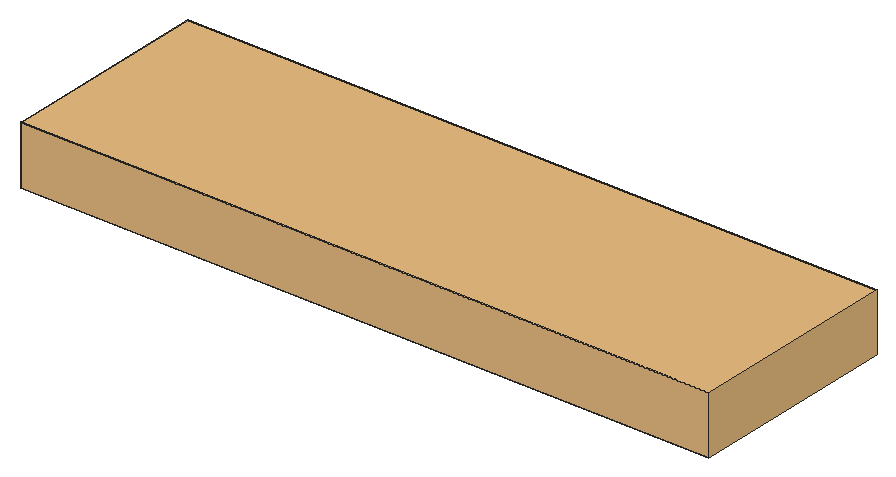
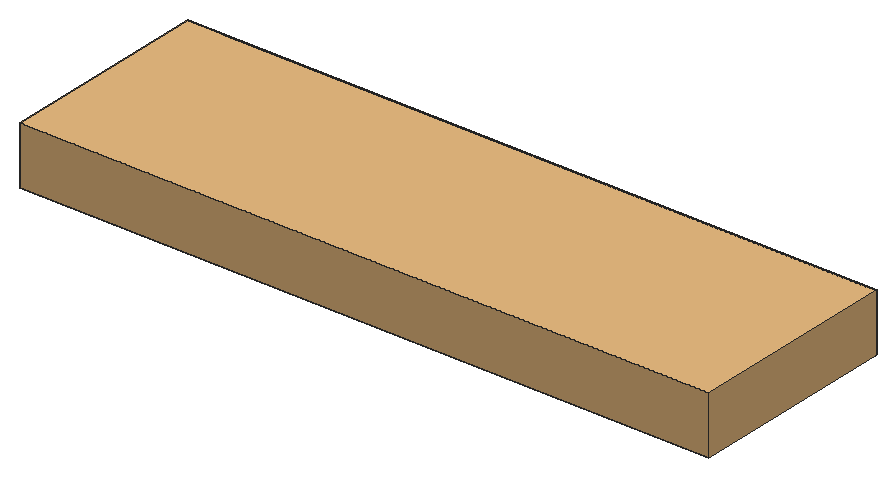
# SketchUp Ruby script. Lengths in inches.
U = 1.inch
M = Sketchup.active_model
def pt(a) = Geom::Point3d.new(a.map { |v| v * U })
def face(e, loops, mat)
  f = e.add_face(loops[0].map { |a| pt(a) })
  loops[1..].each { |l| e.add_face(l.map { |a| pt(a) }).erase! }
  f.material = f.back_material = mat if mat
  f
end
# faces: each face lists its corners as indices into pts; further lists are holes
def faces(e, pts, list, mat = nil) = list.each { |f| face(e, (f[0].is_a?(Array) ? f : [f]).map { |l| l.map { |i| pts[i] } }, mat) }
# xy, xz, yz: faces in a plane at the given z, y or x. An outline is a flat list of corners, or four numbers for a rectangle; further outlines are holes
def ring(l) = l.size == 4 ? [[l[0], l[1]], [l[2], l[1]], [l[2], l[3]], [l[0], l[3]]] : l.each_slice(2).to_a
def flat(e, list, mat, &to3) = list.each { |f| face(e, (f[0].is_a?(Array) ? f : [f]).map { |l| ring(l).map { |u, v| to3.(u, v) } }, mat) }
def xy(e, z, list, mat = nil) = flat(e, list, mat) { |x, y| [x, y, z] }
def xz(e, y, list, mat = nil) = flat(e, list, mat) { |x, z| [x, y, z] }
def yz(e, x, list, mat = nil) = flat(e, list, mat) { |y, z| [x, y, z] }
def lines(e, pts, list) = list.each { |a, b| e.add_line(pt(pts[a]), pt(pts[b])) }
# prism: a flat outline (further loops are holes) pulled along v
def prism(e, loops, v, mat = nil)
  f = face(e, loops, mat); d = Geom::Vector3d.new(v.map { |x| x * U })
  f.pushpull(f.normal.samedirection?(d) ? d.length : -d.length)
end
def box(e, o, s, mat = nil) = prism(e, [[o, [o[0] + s[0], o[1], o[2]], [o[0] + s[0], o[1] + s[1], o[2]], [o[0], o[1] + s[1], o[2]]]], [0, 0, s[2]], mat)
def at(x, y, z, deg = 0) = Geom::Transformation.translation(pt([x, y, z])) * Geom::Transformation.rotation(ORIGIN, Z_AXIS, deg.degrees)
def axes(o, x, y, z) = Geom::Transformation.new([*x, 0, *y, 0, *z, 0, *pt(o).to_a, 1])
def part(name) = M.definitions.add(name)
# library, detail: a bought-in or finely detailed component or shape, given as its bounding box
def library(name, o, s) = part(name).tap { |d| box(d.entities, o, s) }
def detail(e, o, s) = box(e.add_group.entities, o, s)
def put(e, d, t, mat = nil) = e.add_instance(d, t).tap { |i| i.material = mat if mat }
def group(e, t, mat = nil) = e.add_group.tap { |g| g.transformation = t; g.material = mat if mat }.entities
root = M.entities
M.materials.add("False ceiling Light").color = [253, 207, 127]
c1 = library("Group\#34",[0,0,-0.5],[272,74,0.5])
c2 = library("Group\#33",[0,-0.25,0],[284.26,86.25,24])
xz(root,214,[[99,228,368.95,252]])
xz(root,220,[[105,228,368.62,228.5]])
xz(root,221,[[106,228,368.56,228.5]])
xz(root,254,[[240.84,228,240.92,231],[240.92,228,241,231],[241,228,241.08,231],[241.08,228,241.16,231]])
xz(root,260,[[240.84,228,240.92,231],[240.92,228,241,231],[241,228,241.08,231],[241.08,228,241.16,231]])
xz(root,293,[[106,228,376,228.5]])
xz(root,294,[[105,228,377,228.5]])
yz(root,188,[[256.84,228,256.92,231],[256.92,228,257,231],[257,228,257.08,231],[257.08,228,257.16,231]])
yz(root,238,[[256.84,228,256.92,231],[256.92,228,257,231],[257,228,257.08,231],[257.08,228,257.16,231]])
yz(root,244,[[256.84,228,256.92,231],[256.92,228,257,231],[257,228,257.08,231],[257.08,228,257.16,231]])
yz(root,294,[[256.84,228,256.92,231],[256.92,228,257,231],[257,228,257.08,231],[257.08,228,257.16,231]])
p = [[240.53,254.04,228],[240.45,254.05,228],[240.45,254.05,231],[240.53,254.04,231],[240.61,254.03,228],[240.61,254.03,231],
  [240.6875,254.02,228],[240.6875,254.02,231],[240.76,254.01,228],[240.76,254.01,231],[240.84,254,228],[240.84,254,231],
  [241.24,254.01,228],[241.16,254,228],[241.16,254,231],[241.24,254.01,231],[241.3125,254.02,228],[241.3125,254.02,231],
  [241.39,254.03,228],[241.39,254.03,231],[241.47,254.04,228],[241.47,254.04,231],[241.55,254.05,228],[241.55,254.05,231],
  [240.07,254.15,228],[240,254.17,228],[240,254.17,231],[240.07,254.15,231],[240.15,254.125,228],[240.15,254.125,231],
  [240.22,254.1,228],[240.22,254.1,231],[240.3,254.08,228],[240.3,254.08,231],[240.375,254.07,228],[240.375,254.07,231],
  [241.625,254.07,228],[241.625,254.07,231],[241.7,254.08,228],[241.7,254.08,231],[241.78,254.1,228],[241.78,254.1,231],
  [241.85,254.125,228],[241.85,254.125,231],[241.93,254.15,228],[241.93,254.15,231],[242,254.17,228],[242,254.17,231],
  [186.22,254.26,228],[186.15,254.23,228],[186.15,254.23,231],[186.22,254.26,231],[239.85,254.23,228],[239.78,254.26,228],
  [239.78,254.26,231],[239.85,254.23,231],[239.92,254.2,228],[239.92,254.2,231],[242.08,254.2,228],[242.08,254.2,231],
  [242.15,254.23,228],[242.15,254.23,231],[242.22,254.26,228],[242.22,254.26,231],[186.29,254.29,228],[186.29,254.29,231],
  [186.36,254.33,228],[186.36,254.33,231],[186.43,254.36,228],[186.43,254.36,231],[239.64,254.33,228],[239.57,254.36,228],
  [239.57,254.36,231],[239.64,254.33,231],[239.71,254.29,228],[239.71,254.29,231],[242.29,254.29,228],[242.29,254.29,231],
  [242.36,254.33,228],[242.36,254.33,231],[242.43,254.36,228],[242.43,254.36,231],[186.5,254.4,228],[186.5,254.4,231],
  [186.57,254.44,228],[186.57,254.44,231],[186.63,254.48,228],[186.63,254.48,231],[239.43,254.44,228],[239.37,254.48,228],
  [239.37,254.48,231],[239.43,254.44,231],[239.5,254.4,228],[239.5,254.4,231],[242.5,254.4,228],[242.5,254.4,231],
  [242.57,254.44,228],[242.57,254.44,231],[242.63,254.48,228],[242.63,254.48,231],[186.7,254.53,228],[186.7,254.53,231],
  [186.76,254.57,228],[186.76,254.57,231],[239.3,254.53,228],[239.24,254.57,228],[239.24,254.57,231],[239.3,254.53,231],
  [242.7,254.53,228],[242.7,254.53,231],[242.76,254.57,228],[242.76,254.57,231],[186.83,254.62,228],[186.83,254.62,231],
  [186.89,254.67,228],[186.89,254.67,231],[239.17,254.62,228],[239.11,254.67,228],[239.11,254.67,231],[239.17,254.62,231],
  [242.83,254.62,228],[242.83,254.62,231],[242.89,254.67,228],[242.89,254.67,231],[186.95,254.72,228],[186.95,254.72,231],
  [187.01,254.77,228],[187.01,254.77,231],[239.05,254.72,228],[238.99,254.77,228],[238.99,254.77,231],[239.05,254.72,231],
  [242.95,254.72,228],[242.95,254.72,231],[243.01,254.77,228],[243.01,254.77,231],[187.07,254.82,228],[187.07,254.82,231],
  [187.12,254.88,228],[187.12,254.88,231],[238.93,254.82,228],[238.88,254.88,228],[238.88,254.88,231],[238.93,254.82,231],
  [243.07,254.82,228],[243.07,254.82,231],[243.12,254.88,228],[243.12,254.88,231],[187.18,254.93,228],[187.18,254.93,231],
  [187.23,254.99,228],[187.23,254.99,231],[238.82,254.93,228],[238.77,254.99,228],[238.77,254.99,231],[238.82,254.93,231],
  [243.18,254.93,228],[243.18,254.93,231],[243.23,254.99,228],[243.23,254.99,231],[187.28,255.05,228],[187.28,255.05,231],
  [238.72,255.05,228],[238.72,255.05,231],[243.28,255.05,228],[243.28,255.05,231],[294.77,254.99,228],[294.72,255.05,228],
  [294.72,255.05,231],[294.77,254.99,231],[187.33,255.11,228],[187.33,255.11,231],[187.38,255.17,228],[187.38,255.17,231],
  [238.67,255.11,228],[238.62,255.17,228],[238.62,255.17,231],[238.67,255.11,231],[243.33,255.11,228],[243.33,255.11,231],
  [243.38,255.17,228],[243.38,255.17,231],[294.67,255.11,228],[294.62,255.17,228],[294.62,255.17,231],[294.67,255.11,231],
  [187.43,255.24,228],[187.43,255.24,231],[187.47,255.3,228],[187.47,255.3,231],[238.57,255.24,228],[238.53,255.3,228],
  [238.53,255.3,231],[238.57,255.24,231],[243.43,255.24,228],[243.43,255.24,231],[243.47,255.3,228],[243.47,255.3,231],
  [294.57,255.24,228],[294.53,255.3,228],[294.53,255.3,231],[294.57,255.24,231],[187.52,255.37,228],[187.52,255.37,231],
  [238.48,255.37,228],[238.48,255.37,231],[243.52,255.37,228],[243.52,255.37,231],[294.48,255.37,228],[294.48,255.37,231],
  [187.56,255.43,228],[187.56,255.43,231],[187.6,255.5,228],[187.6,255.5,231],[238.44,255.43,228],[238.4,255.5,228],
  [238.4,255.5,231],[238.44,255.43,231],[243.56,255.43,228],[243.56,255.43,231],[243.6,255.5,228],[243.6,255.5,231],
  [294.44,255.43,228],[294.4,255.5,228],[294.4,255.5,231],[294.44,255.43,231],[187.64,255.57,228],[187.64,255.57,231],
  [238.36,255.57,228],[238.36,255.57,231],[243.64,255.57,228],[243.64,255.57,231],[294.36,255.57,228],[294.36,255.57,231],
  [187.67,255.64,228],[187.67,255.64,231],[187.71,255.71,228],[187.71,255.71,231],[238.33,255.64,228],[238.29,255.71,228],
  [238.29,255.71,231],[238.33,255.64,231],[243.67,255.64,228],[243.67,255.64,231],[243.71,255.71,228],[243.71,255.71,231],
  [294.33,255.64,228],[294.29,255.71,228],[294.29,255.71,231],[294.33,255.64,231],[187.74,255.78,228],[187.74,255.78,231],
  [238.26,255.78,228],[238.26,255.78,231],[243.74,255.78,228],[243.74,255.78,231],[294.26,255.78,228],[294.26,255.78,231],
  [187.77,255.85,228],[187.77,255.85,231],[238.23,255.85,228],[238.23,255.85,231],[243.77,255.85,228],[243.77,255.85,231],
  [294.23,255.85,228],[294.23,255.85,231],[187.8,255.92,228],[187.8,255.92,231],[187.83,256,228],[187.83,256,231],
  [238.2,255.92,228],[238.17,256,228],[238.17,256,231],[238.2,255.92,231],[243.8,255.92,228],[243.8,255.92,231],
  [243.83,256,228],[243.83,256,231],[294.2,255.92,228],[294.17,256,228],[294.17,256,231],[294.2,255.92,231],
  [187.85,256.07,228],[187.85,256.07,231],[238.15,256.07,228],[238.15,256.07,231],[243.85,256.07,228],[243.85,256.07,231],
  [294.15,256.07,228],[294.15,256.07,231],[187.875,256.15,228],[187.875,256.15,231],[187.9,256.22,228],[187.9,256.22,231],
  [238.125,256.15,228],[238.1,256.22,228],[238.1,256.22,231],[238.125,256.15,231],[243.875,256.15,228],[243.875,256.15,231],
  [243.9,256.22,228],[243.9,256.22,231],[294.125,256.15,228],[294.1,256.22,228],[294.1,256.22,231],[294.125,256.15,231],
  [187.92,256.3,228],[187.92,256.3,231],[238.08,256.3,228],[238.08,256.3,231],[243.92,256.3,228],[243.92,256.3,231],
  [294.08,256.3,228],[294.08,256.3,231],[187.93,256.375,228],[187.93,256.375,231],[238.07,256.375,228],[238.07,256.375,231],
  [243.93,256.375,228],[243.93,256.375,231],[294.07,256.375,228],[294.07,256.375,231],[187.95,256.45,228],[187.95,256.45,231],
  [238.05,256.45,228],[238.05,256.45,231],[243.95,256.45,228],[243.95,256.45,231],[294.05,256.45,228],[294.05,256.45,231],
  [187.96,256.53,228],[187.96,256.53,231],[187.97,256.61,228],[187.97,256.61,231],[238.04,256.53,228],[238.03,256.61,228],
  [238.03,256.61,231],[238.04,256.53,231],[243.96,256.53,228],[243.96,256.53,231],[243.97,256.61,228],[243.97,256.61,231],
  [294.04,256.53,228],[294.03,256.61,228],[294.03,256.61,231],[294.04,256.53,231],[187.98,256.6875,228],[187.98,256.6875,231],
  [238.02,256.6875,228],[238.02,256.6875,231],[243.98,256.6875,228],[243.98,256.6875,231],[294.02,256.6875,228],[294.02,256.6875,231],
  [187.99,256.76,228],[187.99,256.76,231],[238.01,256.76,228],[238.01,256.76,231],[243.99,256.76,228],[243.99,256.76,231],
  [294.01,256.76,228],[294.01,256.76,231],[188,256.84,228],[188,256.84,231],[238,256.84,228],[238,256.84,231],
  [244,256.84,228],[244,256.84,231],[294,256.84,228],[294,256.84,231],[187.98,257.3125,228],[187.99,257.24,228],
  [187.99,257.24,231],[187.98,257.3125,231],[188,257.16,228],[188,257.16,231],[238,257.16,228],[238.01,257.24,228],
  [238.01,257.24,231],[238,257.16,231],[238.02,257.3125,228],[238.02,257.3125,231],[243.98,257.3125,228],[243.99,257.24,228],
  [243.99,257.24,231],[243.98,257.3125,231],[244,257.16,228],[244,257.16,231],[294,257.16,228],[294.01,257.24,228],
  [294.01,257.24,231],[294,257.16,231],[294.02,257.3125,228],[294.02,257.3125,231],[187.97,257.39,228],[187.97,257.39,231],
  [238.03,257.39,228],[238.03,257.39,231],[243.97,257.39,228],[243.97,257.39,231],[294.03,257.39,228],[294.03,257.39,231],
  [187.96,257.47,228],[187.96,257.47,231],[238.04,257.47,228],[238.04,257.47,231],[243.96,257.47,228],[243.96,257.47,231],
  [294.04,257.47,228],[294.04,257.47,231],[187.93,257.625,228],[187.95,257.55,228],[187.95,257.55,231],[187.93,257.625,231],
  [238.05,257.55,228],[238.05,257.55,231],[238.07,257.625,228],[238.07,257.625,231],[243.93,257.625,228],[243.95,257.55,228],
  [243.95,257.55,231],[243.93,257.625,231],[294.05,257.55,228],[294.05,257.55,231],[294.07,257.625,228],[294.07,257.625,231],
  [187.92,257.7,228],[187.92,257.7,231],[238.08,257.7,228],[238.08,257.7,231],[243.92,257.7,228],[243.92,257.7,231],
  [294.08,257.7,228],[294.08,257.7,231],[187.9,257.78,228],[187.9,257.78,231],[238.1,257.78,228],[238.1,257.78,231],
  [243.9,257.78,228],[243.9,257.78,231],[294.1,257.78,228],[294.1,257.78,231],[187.875,257.85,228],[187.875,257.85,231],
  [238.125,257.85,228],[238.125,257.85,231],[243.875,257.85,228],[243.875,257.85,231],[294.125,257.85,228],[294.125,257.85,231],
  [187.83,258,228],[187.85,257.93,228],[187.85,257.93,231],[187.83,258,231],[238.15,257.93,228],[238.15,257.93,231],
  [238.17,258,228],[238.17,258,231],[243.83,258,228],[243.85,257.93,228],[243.85,257.93,231],[243.83,258,231],
  [294.15,257.93,228],[294.15,257.93,231],[294.17,258,228],[294.17,258,231],[187.8,258.08,228],[187.8,258.08,231],
  [238.2,258.08,228],[238.2,258.08,231],[243.8,258.08,228],[243.8,258.08,231],[294.2,258.08,228],[294.2,258.08,231],
  [187.74,258.22,228],[187.77,258.15,228],[187.77,258.15,231],[187.74,258.22,231],[238.23,258.15,228],[238.23,258.15,231],
  [238.26,258.22,228],[238.26,258.22,231],[243.74,258.22,228],[243.77,258.15,228],[243.77,258.15,231],[243.74,258.22,231],
  [294.23,258.15,228],[294.23,258.15,231],[294.26,258.22,228],[294.26,258.22,231],[187.71,258.29,228],[187.71,258.29,231],
  [238.29,258.29,228],[238.29,258.29,231],[243.71,258.29,228],[243.71,258.29,231],[294.29,258.29,228],[294.29,258.29,231],
  [187.67,258.36,228],[187.67,258.36,231],[238.33,258.36,228],[238.33,258.36,231],[243.67,258.36,228],[243.67,258.36,231],
  [294.33,258.36,228],[294.33,258.36,231],[187.6,258.5,228],[187.64,258.43,228],[187.64,258.43,231],[187.6,258.5,231],
  [238.36,258.43,228],[238.36,258.43,231],[238.4,258.5,228],[238.4,258.5,231],[243.6,258.5,228],[243.64,258.43,228],
  [243.64,258.43,231],[243.6,258.5,231],[294.36,258.43,228],[294.36,258.43,231],[294.4,258.5,228],[294.4,258.5,231],
  [187.56,258.57,228],[187.56,258.57,231],[238.44,258.57,228],[238.44,258.57,231],[243.56,258.57,228],[243.56,258.57,231],
  [294.44,258.57,228],[294.44,258.57,231],[187.47,258.7,228],[187.52,258.63,228],[187.52,258.63,231],[187.47,258.7,231],
  [238.48,258.63,228],[238.48,258.63,231],[238.53,258.7,228],[238.53,258.7,231],[243.47,258.7,228],[243.52,258.63,228],
  [243.52,258.63,231],[243.47,258.7,231],[294.48,258.63,228],[294.48,258.63,231],[294.53,258.7,228],[294.53,258.7,231],
  [187.43,258.76,228],[187.43,258.76,231],[238.57,258.76,228],[238.57,258.76,231],[243.43,258.76,228],[243.43,258.76,231],
  [294.57,258.76,228],[294.57,258.76,231],[187.33,258.89,228],[187.38,258.83,228],[187.38,258.83,231],[187.33,258.89,231],
  [238.62,258.83,228],[238.62,258.83,231],[238.67,258.89,228],[238.67,258.89,231],[243.33,258.89,228],[243.38,258.83,228],
  [243.38,258.83,231],[243.33,258.89,231],[294.62,258.83,228],[294.62,258.83,231],[294.67,258.89,228],[294.67,258.89,231],
  [187.23,259.01,228],[187.28,258.95,228],[187.28,258.95,231],[187.23,259.01,231],[238.72,258.95,228],[238.72,258.95,231],
  [238.77,259.01,228],[238.77,259.01,231],[243.23,259.01,228],[243.28,258.95,228],[243.28,258.95,231],[243.23,259.01,231],
  [294.72,258.95,228],[294.72,258.95,231],[294.77,259.01,228],[294.77,259.01,231],[187.18,259.07,228],[187.18,259.07,231],
  [238.82,259.07,228],[238.82,259.07,231],[243.18,259.07,228],[243.18,259.07,231],[187.07,259.18,228],[187.12,259.12,228],
  [187.12,259.12,231],[187.07,259.18,231],[238.88,259.12,228],[238.88,259.12,231],[238.93,259.18,228],[238.93,259.18,231],
  [243.07,259.18,228],[243.12,259.12,228],[243.12,259.12,231],[243.07,259.18,231],[186.95,259.28,228],[187.01,259.23,228],
  [187.01,259.23,231],[186.95,259.28,231],[238.99,259.23,228],[238.99,259.23,231],[239.05,259.28,228],[239.05,259.28,231],
  [242.95,259.28,228],[243.01,259.23,228],[243.01,259.23,231],[242.95,259.28,231],[186.83,259.38,228],[186.89,259.33,228],
  [186.89,259.33,231],[186.83,259.38,231],[239.11,259.33,228],[239.11,259.33,231],[239.17,259.38,228],[239.17,259.38,231],
  [242.83,259.38,228],[242.89,259.33,228],[242.89,259.33,231],[242.83,259.38,231],[186.7,259.47,228],[186.76,259.43,228],
  [186.76,259.43,231],[186.7,259.47,231],[239.24,259.43,228],[239.24,259.43,231],[239.3,259.47,228],[239.3,259.47,231],
  [242.7,259.47,228],[242.76,259.43,228],[242.76,259.43,231],[242.7,259.47,231],[186.57,259.56,228],[186.63,259.52,228],
  [186.63,259.52,231],[186.57,259.56,231],[239.37,259.52,228],[239.37,259.52,231],[239.43,259.56,228],[239.43,259.56,231],
  [242.57,259.56,228],[242.63,259.52,228],[242.63,259.52,231],[242.57,259.56,231],[186.36,259.67,228],[186.43,259.64,228],
  [186.43,259.64,231],[186.36,259.67,231],[186.5,259.6,228],[186.5,259.6,231],[239.5,259.6,228],[239.5,259.6,231],
  [239.57,259.64,228],[239.57,259.64,231],[239.64,259.67,228],[239.64,259.67,231],[242.36,259.67,228],[242.43,259.64,228],
  [242.43,259.64,231],[242.36,259.67,231],[242.5,259.6,228],[242.5,259.6,231],[186.15,259.77,228],[186.22,259.74,228],
  [186.22,259.74,231],[186.15,259.77,231],[186.29,259.71,228],[186.29,259.71,231],[239.71,259.71,228],[239.71,259.71,231],
  [239.78,259.74,228],[239.78,259.74,231],[239.85,259.77,228],[239.85,259.77,231],[242.15,259.77,228],[242.22,259.74,228],
  [242.22,259.74,231],[242.15,259.77,231],[242.29,259.71,228],[242.29,259.71,231],[239.92,259.8,228],[239.92,259.8,231],
  [240,259.83,228],[240,259.83,231],[240.07,259.85,228],[240.07,259.85,231],[241.93,259.85,228],[242,259.83,228],
  [242,259.83,231],[241.93,259.85,231],[242.08,259.8,228],[242.08,259.8,231],[240.15,259.875,228],[240.15,259.875,231],
  [240.22,259.9,228],[240.22,259.9,231],[240.3,259.92,228],[240.3,259.92,231],[240.375,259.93,228],[240.375,259.93,231],
  [240.45,259.95,228],[240.45,259.95,231],[240.53,259.96,228],[240.53,259.96,231],[241.47,259.96,228],[241.55,259.95,228],
  [241.55,259.95,231],[241.47,259.96,231],[241.625,259.93,228],[241.625,259.93,231],[241.7,259.92,228],[241.7,259.92,231],
  [241.78,259.9,228],[241.78,259.9,231],[241.85,259.875,228],[241.85,259.875,231],[240.61,259.97,228],[240.61,259.97,231],
  [240.6875,259.98,228],[240.6875,259.98,231],[240.76,259.99,228],[240.76,259.99,231],[240.84,260,228],[240.84,260,231],
  [241.16,260,228],[241.24,259.99,228],[241.24,259.99,231],[241.16,260,231],[241.3125,259.98,228],[241.3125,259.98,231],
  [241.39,259.97,228],[241.39,259.97,231]]
faces(root,p,[[0,1,2,3],[4,0,3,5],[6,4,5,7],[8,6,7,9],[10,8,9,11],[12,13,14,15],[16,12,15,17],[18,16,17,19],
  [20,18,19,21],[22,20,21,23],[24,25,26,27],[28,24,27,29],[30,28,29,31],[32,30,31,33],[34,32,33,35],[1,34,35,2],
  [36,22,23,37],[38,36,37,39],[40,38,39,41],[42,40,41,43],[44,42,43,45],[46,44,45,47],[48,49,50,51],[52,53,54,55],
  [56,52,55,57],[25,56,57,26],[58,46,47,59],[60,58,59,61],[62,60,61,63],[64,48,51,65],[66,64,65,67],[68,66,67,69],
  [70,71,72,73],[74,70,73,75],[53,74,75,54],[76,62,63,77],[78,76,77,79],[80,78,79,81],[82,68,69,83],[84,82,83,85],
  [86,84,85,87],[88,89,90,91],[92,88,91,93],[71,92,93,72],[94,80,81,95],[96,94,95,97],[98,96,97,99],[100,86,87,101],
  [102,100,101,103],[104,105,106,107],[89,104,107,90],[108,98,99,109],[110,108,109,111],[112,102,103,113],[114,112,113,115],[116,117,118,119],
  [105,116,119,106],[120,110,111,121],[122,120,121,123],[124,114,115,125],[126,124,125,127],[128,129,130,131],[117,128,131,118],[132,122,123,133],
  [134,132,133,135],[136,126,127,137],[138,136,137,139],[140,141,142,143],[129,140,143,130],[144,134,135,145],[146,144,145,147],[148,138,139,149],
  [150,148,149,151],[152,153,154,155],[141,152,155,142],[156,146,147,157],[158,156,157,159],[160,150,151,161],[153,162,163,154],[164,158,159,165],
  [166,167,168,169],[170,160,161,171],[172,170,171,173],[174,175,176,177],[162,174,177,163],[178,164,165,179],[180,178,179,181],[182,183,184,185],
  [167,182,185,168],[186,172,173,187],[188,186,187,189],[190,191,192,193],[175,190,193,176],[194,180,181,195],[196,194,195,197],[198,199,200,201],
  [183,198,201,184],[202,188,189,203],[191,204,205,192],[206,196,197,207],[199,208,209,200],[210,202,203,211],[212,210,211,213],[214,215,216,217],
  [204,214,217,205],[218,206,207,219],[220,218,219,221],[222,223,224,225],[208,222,225,209],[226,212,213,227],[215,228,229,216],[230,220,221,231],
  [223,232,233,224],[234,226,227,235],[236,234,235,237],[238,239,240,241],[228,238,241,229],[242,230,231,243],[244,242,243,245],[246,247,248,249],
  [232,246,249,233],[250,236,237,251],[239,252,253,240],[254,244,245,255],[247,256,257,248],[258,250,251,259],[252,260,261,253],[262,254,255,263],
  [256,264,265,257],[266,258,259,267],[268,266,267,269],[270,271,272,273],[260,270,273,261],[274,262,263,275],[276,274,275,277],[278,279,280,281],
  [264,278,281,265],[282,268,269,283],[271,284,285,272],[286,276,277,287],[279,288,289,280],[290,282,283,291],[292,290,291,293],[294,295,296,297],
  [284,294,297,285],[298,286,287,299],[300,298,299,301],[302,303,304,305],[288,302,305,289],[306,292,293,307],[295,308,309,296],[310,300,301,311],
  [303,312,313,304],[314,306,307,315],[308,316,317,309],[318,310,311,319],[312,320,321,313],[322,314,315,323],[316,324,325,317],[326,318,319,327],
  [320,328,329,321],[330,322,323,331],[332,330,331,333],[334,335,336,337],[324,334,337,325],[338,326,327,339],[340,338,339,341],[342,343,344,345],
  [328,342,345,329],[346,332,333,347],[335,348,349,336],[350,340,341,351],[343,352,353,344],[354,346,347,355],[348,356,357,349],[358,350,351,359],
  [352,360,361,353],[362,354,355,363],[356,364,365,357],[366,358,359,367],[360,368,369,361],[370,371,372,373],[371,374,375,372],[376,377,378,379],
  [377,380,381,378],[382,383,384,385],[383,386,387,384],[388,389,390,391],[389,392,393,390],[394,370,373,395],[380,396,397,381],[398,382,385,399],
  [392,400,401,393],[402,394,395,403],[396,404,405,397],[406,398,399,407],[400,408,409,401],[410,411,412,413],[411,402,403,412],[404,414,415,405],
  [414,416,417,415],[418,419,420,421],[419,406,407,420],[408,422,423,409],[422,424,425,423],[426,410,413,427],[416,428,429,417],[430,418,421,431],
  [424,432,433,425],[434,426,427,435],[428,436,437,429],[438,430,431,439],[432,440,441,433],[442,434,435,443],[436,444,445,437],[446,438,439,447],
  [440,448,449,441],[450,451,452,453],[451,442,443,452],[444,454,455,445],[454,456,457,455],[458,459,460,461],[459,446,447,460],[448,462,463,449],
  [462,464,465,463],[466,450,453,467],[456,468,469,457],[470,458,461,471],[464,472,473,465],[474,475,476,477],[475,466,467,476],[468,478,479,469],
  [478,480,481,479],[482,483,484,485],[483,470,471,484],[472,486,487,473],[486,488,489,487],[490,474,477,491],[480,492,493,481],[494,482,485,495],
  [488,496,497,489],[498,490,491,499],[492,500,501,493],[502,494,495,503],[496,504,505,497],[506,507,508,509],[507,498,499,508],[500,510,511,501],
  [510,512,513,511],[514,515,516,517],[515,502,503,516],[504,518,519,505],[518,520,521,519],[522,506,509,523],[512,524,525,513],[526,514,517,527],
  [520,528,529,521],[530,531,532,533],[531,522,523,532],[524,534,535,525],[534,536,537,535],[538,539,540,541],[539,526,527,540],[528,542,543,529],
  [542,544,545,543],[546,530,533,547],[536,548,549,537],[550,538,541,551],[544,552,553,545],[554,555,556,557],[555,546,547,556],[548,558,559,549],
  [558,560,561,559],[562,563,564,565],[563,550,551,564],[552,566,567,553],[566,568,569,567],[570,571,572,573],[571,554,557,572],[560,574,575,561],
  [574,576,577,575],[578,579,580,581],[579,562,565,580],[568,582,583,569],[582,584,585,583],[586,570,573,587],[576,588,589,577],[590,578,581,591],
  [592,593,594,595],[593,586,587,594],[588,596,597,589],[596,598,599,597],[600,601,602,603],[601,590,591,602],[604,605,606,607],[605,592,595,606],
  [598,608,609,599],[608,610,611,609],[612,613,614,615],[613,600,603,614],[616,617,618,619],[617,604,607,618],[610,620,621,611],[620,622,623,621],
  [624,625,626,627],[625,612,615,626],[628,629,630,631],[629,616,619,630],[622,632,633,623],[632,634,635,633],[636,637,638,639],[637,624,627,638],
  [640,641,642,643],[641,628,631,642],[634,644,645,635],[644,646,647,645],[648,649,650,651],[649,636,639,650],[652,653,654,655],[653,656,657,654],
  [656,640,643,657],[646,658,659,647],[658,660,661,659],[660,662,663,661],[664,665,666,667],[665,668,669,666],[668,648,651,669],[670,671,672,673],
  [671,674,675,672],[674,652,655,675],[662,676,677,663],[676,678,679,677],[678,680,681,679],[682,683,684,685],[683,686,687,684],[686,664,667,687],
  [680,688,689,681],[688,690,691,689],[690,692,693,691],[694,695,696,697],[695,698,699,696],[698,682,685,699],[692,700,701,693],[700,702,703,701],
  [702,704,705,703],[704,706,707,705],[706,708,709,707],[708,710,711,709],[712,713,714,715],[713,716,717,714],[716,718,719,717],[718,720,721,719],
  [720,722,723,721],[722,694,697,723],[710,724,725,711],[724,726,727,725],[726,728,729,727],[728,730,731,729],[732,733,734,735],[733,736,737,734],
  [736,738,739,737],[738,712,715,739]])
put(root,c1,at(105,220,228.5),"False ceiling Light")
put(root,c2,at(99,214,228))
